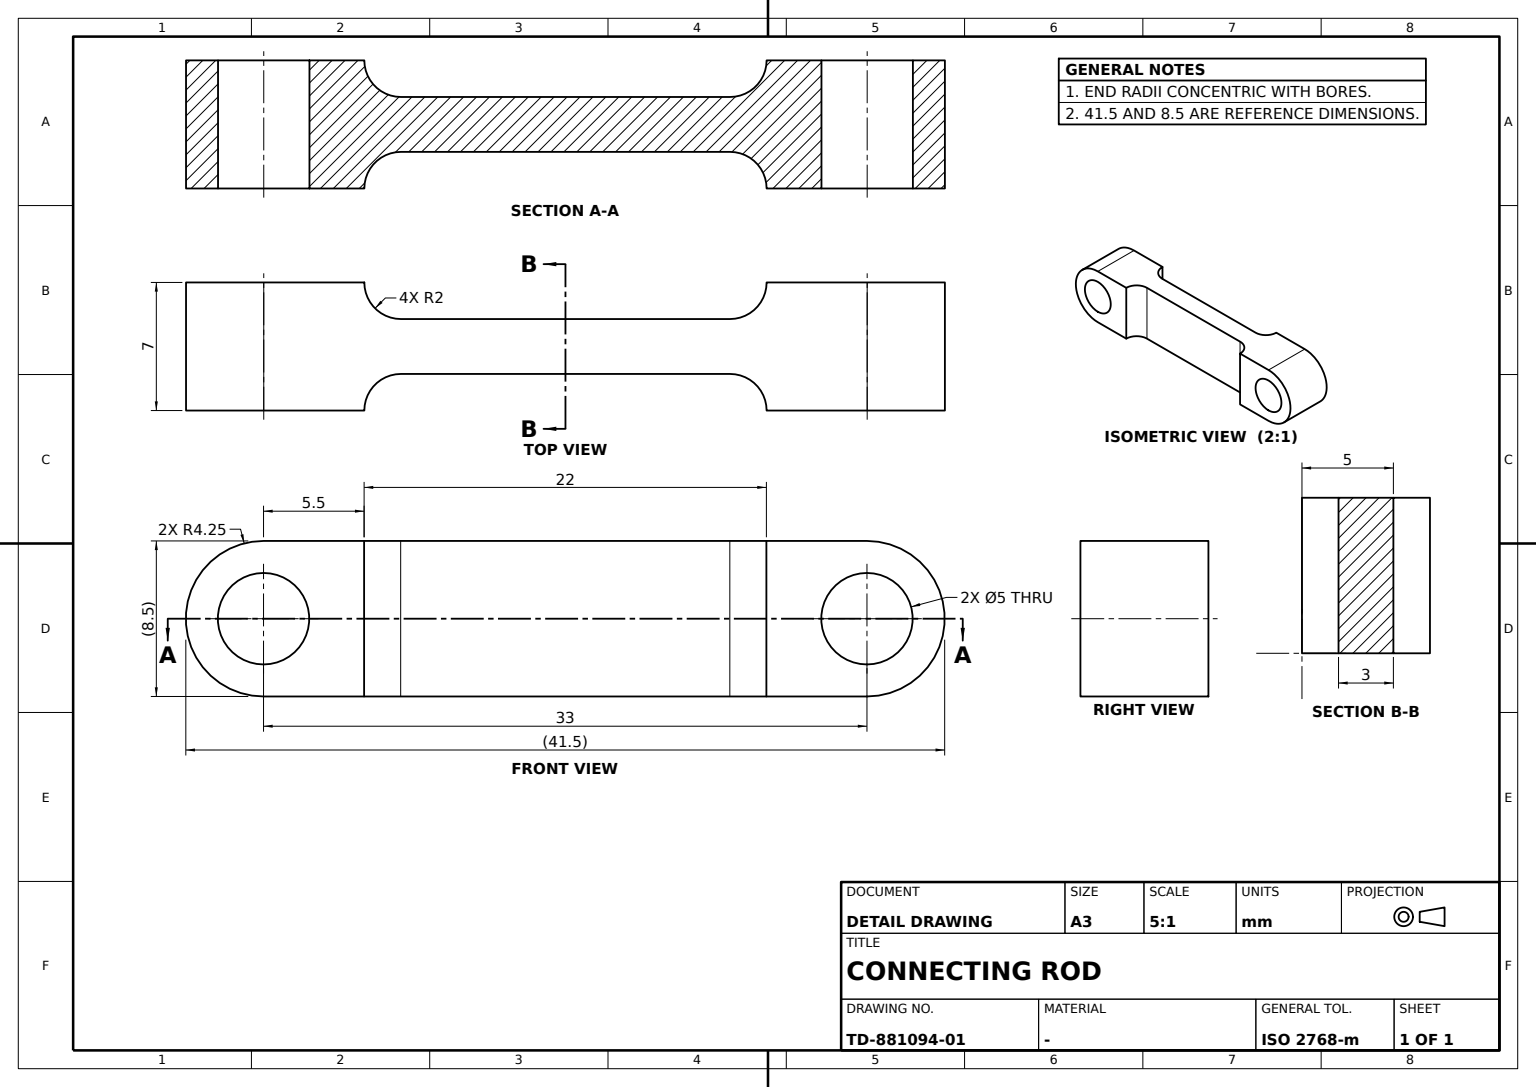
ISO-10303-21;
HEADER;
FILE_DESCRIPTION((''),'2;1');
FILE_NAME('','',(''),(''),'','','');
FILE_SCHEMA(('AUTOMOTIVE_DESIGN'));
ENDSEC;
DATA;
#1=APPLICATION_CONTEXT('');
#2=PRODUCT_CONTEXT('',#1,'mechanical');
#3=PRODUCT('','','',(#2));
#4=PRODUCT_DEFINITION_FORMATION('','',#3);
#5=PRODUCT_DEFINITION_CONTEXT('',#1,'design');
#6=PRODUCT_DEFINITION('','',#4,#5);
#7=PRODUCT_DEFINITION_SHAPE('','',#6);
#8=(LENGTH_UNIT()NAMED_UNIT(*)SI_UNIT(.MILLI.,.METRE.));
#9=(NAMED_UNIT(*)PLANE_ANGLE_UNIT()SI_UNIT($,.RADIAN.));
#10=(NAMED_UNIT(*)SI_UNIT($,.STERADIAN.)SOLID_ANGLE_UNIT());
#11=UNCERTAINTY_MEASURE_WITH_UNIT(LENGTH_MEASURE(0.005),#8,'distance_accuracy_value','');
#12=(GEOMETRIC_REPRESENTATION_CONTEXT(3)GLOBAL_UNCERTAINTY_ASSIGNED_CONTEXT((#11))GLOBAL_UNIT_ASSIGNED_CONTEXT((#8,#9,#10))REPRESENTATION_CONTEXT('',''));
#13=CARTESIAN_POINT('',(-4.25,-16.5,3.5));
#14=VERTEX_POINT('',#13);
#15=CARTESIAN_POINT('',(-4.25,-11.,3.5));
#16=VERTEX_POINT('',#15);
#17=CARTESIAN_POINT('',(-4.25,-11.5,3.5));
#18=DIRECTION('',(0.,1.,0.));
#19=VECTOR('',#18,1000.);
#20=LINE('',#17,#19);
#21=EDGE_CURVE('',#14,#16,#20,.T.);
#22=ORIENTED_EDGE('',*,*,#21,.T.);
#23=CARTESIAN_POINT('',(-4.25,-9.,1.5));
#24=VERTEX_POINT('',#23);
#25=CARTESIAN_POINT('',(-4.25,-9.,3.5));
#26=DIRECTION('',(-1.,0.,0.));
#27=DIRECTION('',(0.,0.,1.));
#28=AXIS2_PLACEMENT_3D('',#25,#26,#27);
#29=CIRCLE('',#28,2.);
#30=EDGE_CURVE('',#24,#16,#29,.T.);
#31=ORIENTED_EDGE('',*,*,#30,.F.);
#32=CARTESIAN_POINT('',(-4.25,9.,1.5));
#33=VERTEX_POINT('',#32);
#34=CARTESIAN_POINT('',(-4.25,-11.5,1.5));
#35=DIRECTION('',(0.,-1.,0.));
#36=VECTOR('',#35,1000.);
#37=LINE('',#34,#36);
#38=EDGE_CURVE('',#33,#24,#37,.T.);
#39=ORIENTED_EDGE('',*,*,#38,.F.);
#40=CARTESIAN_POINT('',(-4.25,11.,3.5));
#41=VERTEX_POINT('',#40);
#42=CARTESIAN_POINT('',(-4.25,9.,3.5));
#43=AXIS2_PLACEMENT_3D('',#42,#26,#27);
#44=CIRCLE('',#43,2.);
#45=EDGE_CURVE('',#41,#33,#44,.T.);
#46=ORIENTED_EDGE('',*,*,#45,.F.);
#47=CARTESIAN_POINT('',(-4.25,16.5,3.5));
#48=VERTEX_POINT('',#47);
#49=EDGE_CURVE('',#41,#48,#20,.T.);
#50=ORIENTED_EDGE('',*,*,#49,.T.);
#51=CARTESIAN_POINT('',(-4.25,16.5,-3.5));
#52=VERTEX_POINT('',#51);
#53=CARTESIAN_POINT('',(-4.25,16.5,0.));
#54=VECTOR('',#27,1000.);
#55=LINE('',#53,#54);
#56=EDGE_CURVE('',#52,#48,#55,.T.);
#57=ORIENTED_EDGE('',*,*,#56,.F.);
#58=CARTESIAN_POINT('',(-4.25,11.,-3.5));
#59=VERTEX_POINT('',#58);
#60=CARTESIAN_POINT('',(-4.25,-11.5,-3.5));
#61=LINE('',#60,#19);
#62=EDGE_CURVE('',#52,#59,#61,.F.);
#63=ORIENTED_EDGE('',*,*,#62,.T.);
#64=CARTESIAN_POINT('',(-4.25,9.,-1.5));
#65=VERTEX_POINT('',#64);
#66=CARTESIAN_POINT('',(-4.25,9.,-3.5));
#67=AXIS2_PLACEMENT_3D('',#66,#26,#27);
#68=CIRCLE('',#67,2.);
#69=EDGE_CURVE('',#65,#59,#68,.T.);
#70=ORIENTED_EDGE('',*,*,#69,.F.);
#71=CARTESIAN_POINT('',(-4.25,-9.,-1.5));
#72=VERTEX_POINT('',#71);
#73=CARTESIAN_POINT('',(-4.25,-11.5,-1.5));
#74=LINE('',#73,#36);
#75=EDGE_CURVE('',#65,#72,#74,.T.);
#76=ORIENTED_EDGE('',*,*,#75,.T.);
#77=CARTESIAN_POINT('',(-4.25,-11.,-3.5));
#78=VERTEX_POINT('',#77);
#79=CARTESIAN_POINT('',(-4.25,-9.,-3.5));
#80=AXIS2_PLACEMENT_3D('',#79,#26,#27);
#81=CIRCLE('',#80,2.);
#82=EDGE_CURVE('',#78,#72,#81,.T.);
#83=ORIENTED_EDGE('',*,*,#82,.F.);
#84=CARTESIAN_POINT('',(-4.25,-16.5,-3.5));
#85=VERTEX_POINT('',#84);
#86=CARTESIAN_POINT('',(-4.25,0.,-3.5));
#87=LINE('',#86,#36);
#88=EDGE_CURVE('',#78,#85,#87,.T.);
#89=ORIENTED_EDGE('',*,*,#88,.T.);
#90=CARTESIAN_POINT('',(-4.25,-16.5,0.));
#91=LINE('',#90,#54);
#92=EDGE_CURVE('',#85,#14,#91,.T.);
#93=ORIENTED_EDGE('',*,*,#92,.T.);
#94=EDGE_LOOP('',(#22,#31,#39,#46,#50,#57,#63,#70,#76,#83,#89,#93));
#95=FACE_BOUND('',#94,.T.);
#96=CARTESIAN_POINT('',(-4.25,-11.5,0.));
#97=AXIS2_PLACEMENT_3D('',#96,#26,#35);
#98=PLANE('',#97);
#99=ADVANCED_FACE('',(#95),#98,.T.);
#100=CARTESIAN_POINT('',(4.25,16.5,3.5));
#101=VERTEX_POINT('',#100);
#102=CARTESIAN_POINT('',(0.,16.5,3.5));
#103=DIRECTION('',(1.,0.,0.));
#104=AXIS2_PLACEMENT_3D('',#102,#27,#103);
#105=CIRCLE('',#104,4.25);
#106=EDGE_CURVE('',#101,#48,#105,.T.);
#107=ORIENTED_EDGE('',*,*,#106,.T.);
#108=ORIENTED_EDGE('',*,*,#49,.F.);
#109=CARTESIAN_POINT('',(4.25,11.,3.5));
#110=VERTEX_POINT('',#109);
#111=VECTOR('',#26,1000.);
#112=LINE('',#109,#111);
#113=EDGE_CURVE('',#110,#41,#112,.T.);
#114=ORIENTED_EDGE('',*,*,#113,.F.);
#115=CARTESIAN_POINT('',(4.25,-16.5,3.5));
#116=LINE('',#115,#36);
#117=EDGE_CURVE('',#110,#101,#116,.F.);
#118=ORIENTED_EDGE('',*,*,#117,.T.);
#119=EDGE_LOOP('',(#107,#108,#114,#118));
#120=FACE_BOUND('',#119,.T.);
#121=CARTESIAN_POINT('',(2.5,16.5,3.5));
#122=VERTEX_POINT('',#121);
#123=CIRCLE('',#104,2.5);
#124=EDGE_CURVE('',#122,#122,#123,.T.);
#125=ORIENTED_EDGE('',*,*,#124,.F.);
#126=EDGE_LOOP('',(#125));
#127=FACE_BOUND('',#126,.T.);
#128=CARTESIAN_POINT('',(0.,0.,3.5));
#129=AXIS2_PLACEMENT_3D('',#128,#27,#18);
#130=PLANE('',#129);
#131=ADVANCED_FACE('',(#120,#127),#130,.T.);
#132=CARTESIAN_POINT('',(4.25,-11.,3.5));
#133=VERTEX_POINT('',#132);
#134=LINE('',#132,#111);
#135=EDGE_CURVE('',#133,#16,#134,.T.);
#136=ORIENTED_EDGE('',*,*,#135,.F.);
#137=CARTESIAN_POINT('',(4.25,-9.,1.5));
#138=VERTEX_POINT('',#137);
#139=CARTESIAN_POINT('',(4.25,-9.,3.5));
#140=DIRECTION('',(0.,0.,-1.));
#141=AXIS2_PLACEMENT_3D('',#139,#103,#140);
#142=CIRCLE('',#141,2.);
#143=EDGE_CURVE('',#133,#138,#142,.T.);
#144=ORIENTED_EDGE('',*,*,#143,.T.);
#145=CARTESIAN_POINT('',(0.,-9.,1.5));
#146=LINE('',#145,#111);
#147=EDGE_CURVE('',#138,#24,#146,.T.);
#148=ORIENTED_EDGE('',*,*,#147,.T.);
#149=ORIENTED_EDGE('',*,*,#30,.T.);
#150=EDGE_LOOP('',(#136,#144,#148,#149));
#151=FACE_BOUND('',#150,.T.);
#152=CARTESIAN_POINT('',(0.,-9.,3.5));
#153=AXIS2_PLACEMENT_3D('',#152,#26,#140);
#154=CYLINDRICAL_SURFACE('',#153,2.);
#155=ADVANCED_FACE('',(#151),#154,.F.);
#156=CARTESIAN_POINT('',(4.25,9.,-1.5));
#157=VERTEX_POINT('',#156);
#158=CARTESIAN_POINT('',(0.,9.,-1.5));
#159=LINE('',#158,#111);
#160=EDGE_CURVE('',#157,#65,#159,.T.);
#161=ORIENTED_EDGE('',*,*,#160,.F.);
#162=CARTESIAN_POINT('',(4.25,-9.,-1.5));
#163=VERTEX_POINT('',#162);
#164=CARTESIAN_POINT('',(4.25,11.,-1.5));
#165=LINE('',#164,#36);
#166=EDGE_CURVE('',#157,#163,#165,.T.);
#167=ORIENTED_EDGE('',*,*,#166,.T.);
#168=CARTESIAN_POINT('',(0.,-9.,-1.5));
#169=LINE('',#168,#111);
#170=EDGE_CURVE('',#163,#72,#169,.T.);
#171=ORIENTED_EDGE('',*,*,#170,.T.);
#172=ORIENTED_EDGE('',*,*,#75,.F.);
#173=EDGE_LOOP('',(#161,#167,#171,#172));
#174=FACE_BOUND('',#173,.T.);
#175=AXIS2_PLACEMENT_3D('',#164,#140,#35);
#176=PLANE('',#175);
#177=ADVANCED_FACE('',(#174),#176,.T.);
#178=ORIENTED_EDGE('',*,*,#45,.T.);
#179=CARTESIAN_POINT('',(4.25,9.,1.5));
#180=VERTEX_POINT('',#179);
#181=CARTESIAN_POINT('',(0.,9.,1.5));
#182=LINE('',#181,#111);
#183=EDGE_CURVE('',#180,#33,#182,.T.);
#184=ORIENTED_EDGE('',*,*,#183,.F.);
#185=CARTESIAN_POINT('',(4.25,9.,3.5));
#186=AXIS2_PLACEMENT_3D('',#185,#103,#140);
#187=CIRCLE('',#186,2.);
#188=EDGE_CURVE('',#180,#110,#187,.T.);
#189=ORIENTED_EDGE('',*,*,#188,.T.);
#190=ORIENTED_EDGE('',*,*,#113,.T.);
#191=EDGE_LOOP('',(#178,#184,#189,#190));
#192=FACE_BOUND('',#191,.T.);
#193=CARTESIAN_POINT('',(0.,9.,3.5));
#194=AXIS2_PLACEMENT_3D('',#193,#26,#18);
#195=CYLINDRICAL_SURFACE('',#194,2.);
#196=ADVANCED_FACE('',(#192),#195,.F.);
#197=ORIENTED_EDGE('',*,*,#124,.T.);
#198=EDGE_LOOP('',(#197));
#199=FACE_BOUND('',#198,.T.);
#200=CARTESIAN_POINT('',(2.5,16.5,-3.5));
#201=VERTEX_POINT('',#200);
#202=CARTESIAN_POINT('',(0.,16.5,-3.5));
#203=AXIS2_PLACEMENT_3D('',#202,#27,#103);
#204=CIRCLE('',#203,2.5);
#205=EDGE_CURVE('',#201,#201,#204,.T.);
#206=ORIENTED_EDGE('',*,*,#205,.F.);
#207=EDGE_LOOP('',(#206));
#208=FACE_BOUND('',#207,.T.);
#209=CARTESIAN_POINT('',(0.,16.5,0.));
#210=AXIS2_PLACEMENT_3D('',#209,#27,#18);
#211=CYLINDRICAL_SURFACE('',#210,2.5);
#212=ADVANCED_FACE('',(#199,#208),#211,.F.);
#213=ORIENTED_EDGE('',*,*,#56,.T.);
#214=ORIENTED_EDGE('',*,*,#106,.F.);
#215=CARTESIAN_POINT('',(4.25,16.5,-3.5));
#216=VERTEX_POINT('',#215);
#217=CARTESIAN_POINT('',(4.25,16.5,0.));
#218=LINE('',#217,#54);
#219=EDGE_CURVE('',#216,#101,#218,.T.);
#220=ORIENTED_EDGE('',*,*,#219,.F.);
#221=CIRCLE('',#203,4.25);
#222=EDGE_CURVE('',#216,#52,#221,.T.);
#223=ORIENTED_EDGE('',*,*,#222,.T.);
#224=EDGE_LOOP('',(#213,#214,#220,#223));
#225=FACE_BOUND('',#224,.T.);
#226=CYLINDRICAL_SURFACE('',#210,4.25);
#227=ADVANCED_FACE('',(#225),#226,.T.);
#228=ORIENTED_EDGE('',*,*,#219,.T.);
#229=ORIENTED_EDGE('',*,*,#117,.F.);
#230=ORIENTED_EDGE('',*,*,#188,.F.);
#231=CARTESIAN_POINT('',(4.25,11.,1.5));
#232=LINE('',#231,#36);
#233=EDGE_CURVE('',#180,#138,#232,.T.);
#234=ORIENTED_EDGE('',*,*,#233,.T.);
#235=ORIENTED_EDGE('',*,*,#143,.F.);
#236=VERTEX_POINT('',#115);
#237=CARTESIAN_POINT('',(4.25,0.,3.5));
#238=LINE('',#237,#19);
#239=EDGE_CURVE('',#236,#133,#238,.T.);
#240=ORIENTED_EDGE('',*,*,#239,.F.);
#241=CARTESIAN_POINT('',(4.25,-16.5,-3.5));
#242=VERTEX_POINT('',#241);
#243=CARTESIAN_POINT('',(4.25,-16.5,0.));
#244=LINE('',#243,#54);
#245=EDGE_CURVE('',#242,#236,#244,.T.);
#246=ORIENTED_EDGE('',*,*,#245,.F.);
#247=CARTESIAN_POINT('',(4.25,-11.,-3.5));
#248=VERTEX_POINT('',#247);
#249=CARTESIAN_POINT('',(4.25,0.,-3.5));
#250=LINE('',#249,#19);
#251=EDGE_CURVE('',#248,#242,#250,.F.);
#252=ORIENTED_EDGE('',*,*,#251,.F.);
#253=CARTESIAN_POINT('',(4.25,-9.,-3.5));
#254=AXIS2_PLACEMENT_3D('',#253,#103,#140);
#255=CIRCLE('',#254,2.);
#256=EDGE_CURVE('',#163,#248,#255,.T.);
#257=ORIENTED_EDGE('',*,*,#256,.F.);
#258=ORIENTED_EDGE('',*,*,#166,.F.);
#259=CARTESIAN_POINT('',(4.25,11.,-3.5));
#260=VERTEX_POINT('',#259);
#261=CARTESIAN_POINT('',(4.25,9.,-3.5));
#262=AXIS2_PLACEMENT_3D('',#261,#103,#140);
#263=CIRCLE('',#262,2.);
#264=EDGE_CURVE('',#260,#157,#263,.T.);
#265=ORIENTED_EDGE('',*,*,#264,.F.);
#266=LINE('',#241,#36);
#267=EDGE_CURVE('',#216,#260,#266,.T.);
#268=ORIENTED_EDGE('',*,*,#267,.F.);
#269=EDGE_LOOP('',(#228,#229,#230,#234,#235,#240,#246,#252,#257,#258,#265,#268));
#270=FACE_BOUND('',#269,.T.);
#271=AXIS2_PLACEMENT_3D('',#243,#103,#18);
#272=PLANE('',#271);
#273=ADVANCED_FACE('',(#270),#272,.T.);
#274=CARTESIAN_POINT('',(0.,-16.5,3.5));
#275=AXIS2_PLACEMENT_3D('',#274,#27,#103);
#276=CIRCLE('',#275,4.25);
#277=EDGE_CURVE('',#14,#236,#276,.T.);
#278=ORIENTED_EDGE('',*,*,#277,.F.);
#279=ORIENTED_EDGE('',*,*,#92,.F.);
#280=CARTESIAN_POINT('',(0.,-16.5,-3.5));
#281=AXIS2_PLACEMENT_3D('',#280,#27,#103);
#282=CIRCLE('',#281,4.25);
#283=EDGE_CURVE('',#85,#242,#282,.T.);
#284=ORIENTED_EDGE('',*,*,#283,.T.);
#285=ORIENTED_EDGE('',*,*,#245,.T.);
#286=EDGE_LOOP('',(#278,#279,#284,#285));
#287=FACE_BOUND('',#286,.T.);
#288=CARTESIAN_POINT('',(0.,-16.5,0.));
#289=AXIS2_PLACEMENT_3D('',#288,#27,#18);
#290=CYLINDRICAL_SURFACE('',#289,4.25);
#291=ADVANCED_FACE('',(#287),#290,.T.);
#292=CARTESIAN_POINT('',(2.5,-16.5,-3.5));
#293=VERTEX_POINT('',#292);
#294=CIRCLE('',#281,2.5);
#295=EDGE_CURVE('',#293,#293,#294,.T.);
#296=ORIENTED_EDGE('',*,*,#295,.T.);
#297=EDGE_LOOP('',(#296));
#298=FACE_BOUND('',#297,.T.);
#299=LINE('',#247,#111);
#300=EDGE_CURVE('',#248,#78,#299,.T.);
#301=ORIENTED_EDGE('',*,*,#300,.F.);
#302=ORIENTED_EDGE('',*,*,#251,.T.);
#303=ORIENTED_EDGE('',*,*,#283,.F.);
#304=ORIENTED_EDGE('',*,*,#88,.F.);
#305=EDGE_LOOP('',(#301,#302,#303,#304));
#306=FACE_BOUND('',#305,.T.);
#307=CARTESIAN_POINT('',(0.,0.,-3.5));
#308=AXIS2_PLACEMENT_3D('',#307,#27,#18);
#309=PLANE('',#308);
#310=ADVANCED_FACE('',(#298,#306),#309,.F.);
#311=CARTESIAN_POINT('',(2.5,-16.5,3.5));
#312=VERTEX_POINT('',#311);
#313=CIRCLE('',#275,2.5);
#314=EDGE_CURVE('',#312,#312,#313,.T.);
#315=ORIENTED_EDGE('',*,*,#314,.T.);
#316=EDGE_LOOP('',(#315));
#317=FACE_BOUND('',#316,.T.);
#318=ORIENTED_EDGE('',*,*,#295,.F.);
#319=EDGE_LOOP('',(#318));
#320=FACE_BOUND('',#319,.T.);
#321=CYLINDRICAL_SURFACE('',#289,2.5);
#322=ADVANCED_FACE('',(#317,#320),#321,.F.);
#323=ORIENTED_EDGE('',*,*,#21,.F.);
#324=ORIENTED_EDGE('',*,*,#277,.T.);
#325=ORIENTED_EDGE('',*,*,#239,.T.);
#326=ORIENTED_EDGE('',*,*,#135,.T.);
#327=EDGE_LOOP('',(#323,#324,#325,#326));
#328=FACE_BOUND('',#327,.T.);
#329=ORIENTED_EDGE('',*,*,#314,.F.);
#330=EDGE_LOOP('',(#329));
#331=FACE_BOUND('',#330,.T.);
#332=ADVANCED_FACE('',(#328,#331),#130,.T.);
#333=ORIENTED_EDGE('',*,*,#69,.T.);
#334=LINE('',#259,#111);
#335=EDGE_CURVE('',#260,#59,#334,.T.);
#336=ORIENTED_EDGE('',*,*,#335,.F.);
#337=ORIENTED_EDGE('',*,*,#264,.T.);
#338=ORIENTED_EDGE('',*,*,#160,.T.);
#339=EDGE_LOOP('',(#333,#336,#337,#338));
#340=FACE_BOUND('',#339,.T.);
#341=CARTESIAN_POINT('',(0.,9.,-3.5));
#342=AXIS2_PLACEMENT_3D('',#341,#26,#27);
#343=CYLINDRICAL_SURFACE('',#342,2.);
#344=ADVANCED_FACE('',(#340),#343,.F.);
#345=ORIENTED_EDGE('',*,*,#335,.T.);
#346=ORIENTED_EDGE('',*,*,#62,.F.);
#347=ORIENTED_EDGE('',*,*,#222,.F.);
#348=ORIENTED_EDGE('',*,*,#267,.T.);
#349=EDGE_LOOP('',(#345,#346,#347,#348));
#350=FACE_BOUND('',#349,.T.);
#351=ORIENTED_EDGE('',*,*,#205,.T.);
#352=EDGE_LOOP('',(#351));
#353=FACE_BOUND('',#352,.T.);
#354=ADVANCED_FACE('',(#350,#353),#309,.F.);
#355=ORIENTED_EDGE('',*,*,#300,.T.);
#356=ORIENTED_EDGE('',*,*,#82,.T.);
#357=ORIENTED_EDGE('',*,*,#170,.F.);
#358=ORIENTED_EDGE('',*,*,#256,.T.);
#359=EDGE_LOOP('',(#355,#356,#357,#358));
#360=FACE_BOUND('',#359,.T.);
#361=CARTESIAN_POINT('',(0.,-9.,-3.5));
#362=AXIS2_PLACEMENT_3D('',#361,#26,#35);
#363=CYLINDRICAL_SURFACE('',#362,2.);
#364=ADVANCED_FACE('',(#360),#363,.F.);
#365=ORIENTED_EDGE('',*,*,#233,.F.);
#366=ORIENTED_EDGE('',*,*,#183,.T.);
#367=ORIENTED_EDGE('',*,*,#38,.T.);
#368=ORIENTED_EDGE('',*,*,#147,.F.);
#369=EDGE_LOOP('',(#365,#366,#367,#368));
#370=FACE_BOUND('',#369,.T.);
#371=AXIS2_PLACEMENT_3D('',#231,#140,#35);
#372=PLANE('',#371);
#373=ADVANCED_FACE('',(#370),#372,.F.);
#374=CLOSED_SHELL('',(#99,#131,#155,#177,#196,#212,#227,#273,#291,#310,#322,#332,#344,#354,#364,#373));
#375=MANIFOLD_SOLID_BREP('',#374);
#376=ADVANCED_BREP_SHAPE_REPRESENTATION('',(#375),#12);
#377=SHAPE_DEFINITION_REPRESENTATION(#7,#376);
ENDSEC;
END-ISO-10303-21;
